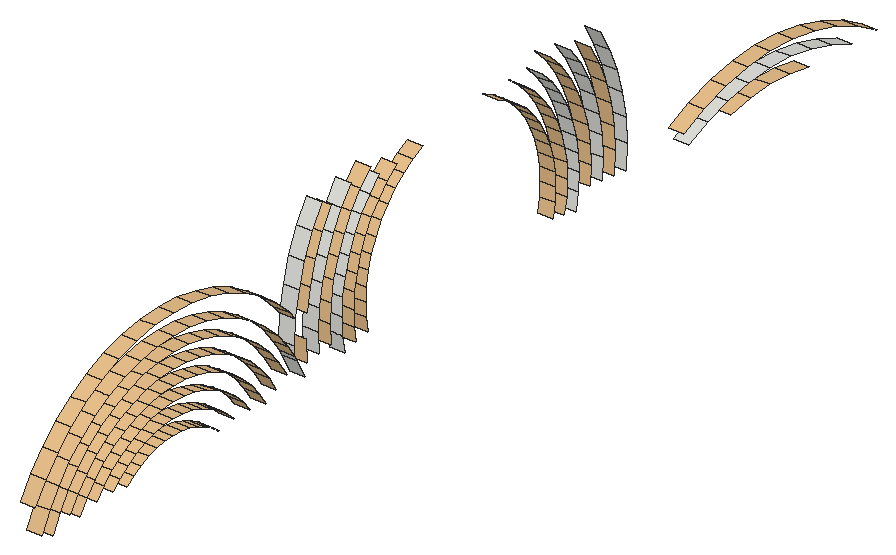
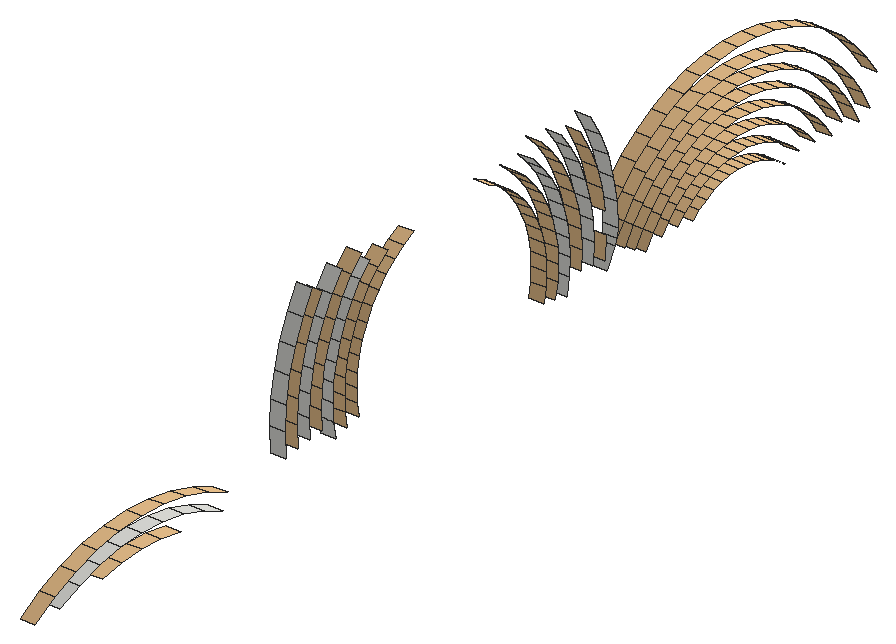
# SketchUp Ruby script. Lengths in inches.
U = 1.inch
M = Sketchup.active_model
def pt(a) = Geom::Point3d.new(a.map { |v| v * U })
def face(e, loops, mat)
  f = e.add_face(loops[0].map { |a| pt(a) })
  loops[1..].each { |l| e.add_face(l.map { |a| pt(a) }).erase! }
  f.material = f.back_material = mat if mat
  f
end
# faces: each face lists its corners as indices into pts; further lists are holes
def faces(e, pts, list, mat = nil) = list.each { |f| face(e, (f[0].is_a?(Array) ? f : [f]).map { |l| l.map { |i| pts[i] } }, mat) }
# xy, xz, yz: faces in a plane at the given z, y or x. An outline is a flat list of corners, or four numbers for a rectangle; further outlines are holes
def ring(l) = l.size == 4 ? [[l[0], l[1]], [l[2], l[1]], [l[2], l[3]], [l[0], l[3]]] : l.each_slice(2).to_a
def flat(e, list, mat, &to3) = list.each { |f| face(e, (f[0].is_a?(Array) ? f : [f]).map { |l| ring(l).map { |u, v| to3.(u, v) } }, mat) }
def xy(e, z, list, mat = nil) = flat(e, list, mat) { |x, y| [x, y, z] }
def xz(e, y, list, mat = nil) = flat(e, list, mat) { |x, z| [x, y, z] }
def yz(e, x, list, mat = nil) = flat(e, list, mat) { |y, z| [x, y, z] }
def lines(e, pts, list) = list.each { |a, b| e.add_line(pt(pts[a]), pt(pts[b])) }
# prism: a flat outline (further loops are holes) pulled along v
def prism(e, loops, v, mat = nil)
  f = face(e, loops, mat); d = Geom::Vector3d.new(v.map { |x| x * U })
  f.pushpull(f.normal.samedirection?(d) ? d.length : -d.length)
end
def box(e, o, s, mat = nil) = prism(e, [[o, [o[0] + s[0], o[1], o[2]], [o[0] + s[0], o[1] + s[1], o[2]], [o[0], o[1] + s[1], o[2]]]], [0, 0, s[2]], mat)
def at(x, y, z, deg = 0) = Geom::Transformation.translation(pt([x, y, z])) * Geom::Transformation.rotation(ORIGIN, Z_AXIS, deg.degrees)
def axes(o, x, y, z) = Geom::Transformation.new([*x, 0, *y, 0, *z, 0, *pt(o).to_a, 1])
def part(name) = M.definitions.add(name)
# library, detail: a bought-in or finely detailed component or shape, given as its bounding box
def library(name, o, s) = part(name).tap { |d| box(d.entities, o, s) }
def detail(e, o, s) = box(e.add_group.entities, o, s)
def put(e, d, t, mat = nil) = e.add_instance(d, t).tap { |i| i.material = mat if mat }
def group(e, t, mat = nil) = e.add_group.tap { |g| g.transformation = t; g.material = mat if mat }.entities
root = M.entities
M.materials.add("images").color = [235, 194, 141]
xz(root,90.53,[[183.82,66.87,185.82,66.88]])
p = [[183.82,51.02,60.88],[183.82,49.86,58.6],[185.82,49.86,58.6],[185.82,51.02,60.88],[183.82,85.65,58.71],[183.82,84.51,60.46],
  [185.82,84.51,60.46],[185.82,85.65,58.71],[183.82,156.61,58.71],[183.82,159.86,60.13],[185.82,159.86,60.13],[185.82,156.61,58.71],
  [183.82,188.1,58.8],[183.82,184.82,60.66],[185.82,184.82,60.66],[185.82,188.1,58.8],[183.82,55.64,60.6],[183.82,54.48,58.86],
  [185.82,54.48,58.86],[185.82,55.64,60.6],[183.82,76.66,59.78],[183.82,77.78,58.9375],[185.82,77.78,58.9375],[185.82,76.66,59.78],
  [183.82,180.68,60.25],[183.82,183.93,58.87],[185.82,183.93,58.87],[185.82,180.68,60.25],[183.82,62.35,59.01],[183.82,63.48,59.84],
  [185.82,63.48,59.84],[185.82,62.35,59.01],[183.82,98.47,61.31],[183.82,98.87,59.03],[185.82,98.87,59.03],[185.82,98.47,61.31],
  [183.82,137.66,58.97],[183.82,138.07,61.25],[185.82,138.07,61.25],[185.82,137.66,58.97],[183.82,90.86,61.68],[183.82,92.1,59.18],
  [185.82,92.1,59.18],[185.82,90.86,61.68],[183.82,166.97,59.8125],[183.82,163.71,59.22],[185.82,163.71,59.22],[185.82,166.97,59.8125],
  [183.82,80.25,59.34],[183.82,79.07,60.46],[185.82,79.07,60.46],[185.82,80.25,59.34],[183.82,81.71,60.71],[183.82,82.9,59.27],
  [185.82,82.9,59.27],[185.82,81.71,60.71],[183.82,176.83,59.3],[183.82,173.57,59.85],[185.82,173.57,59.85],[185.82,176.83,59.3],
  [183.82,48.03,59.4],[183.82,49.3,61.89],[185.82,49.3,61.89],[185.82,48.03,59.4],[183.82,57.23,59.4],[183.82,58.4375,60.82],
  [185.82,58.4375,60.82],[185.82,57.23,59.4],[183.82,61.07,60.55],[183.82,59.88,59.44],[185.82,59.88,59.44],[185.82,61.07,60.55],
  [183.82,136.08,61.49],[183.82,135.72,59.43],[185.82,135.72,59.43],[185.82,136.08,61.49],[183.82,100.8125,59.48],[183.82,100.45,61.54],
  [185.82,100.45,61.54],[185.82,100.8125,59.48],[183.82,86.12,61.65],[183.82,87.39,59.7],[185.82,87.39,59.7],[185.82,86.12,61.65],
  [183.82,64.6875,60.53],[185.82,64.6875,60.53],[183.82,75.46,60.48],[185.82,75.46,60.48],[183.82,170.27,60.03],[185.82,170.27,60.03],
  [183.82,52.75,59.87],[183.82,54.04,61.81],[185.82,54.04,61.81],[185.82,52.75,59.87],[183.82,102.44,61.77],[183.82,102.76,59.94],
  [185.82,102.76,59.94],[185.82,102.44,61.77],[183.82,133.77,59.9],[183.82,134.09,61.72],[185.82,134.09,61.72],[185.82,133.77,59.9],
  [183.82,163.24,61.16],[185.82,163.24,61.16],[183.82,146.01,60.31],[183.82,146.2,63.55],[185.82,146.2,63.55],[185.82,146.01,60.31],
  [183.82,177.28,61.25],[185.82,177.28,61.25],[183.82,65.97,61.08],[185.82,65.97,61.08],[183.82,74.18,61.04],[185.82,74.18,61.04],
  [183.82,77.77,61.44],[185.82,77.77,61.44],[183.82,83.17,62.07],[185.82,83.17,62.07],[183.82,144.2,63.56],[183.82,144.02,60.55],
  [185.82,144.02,60.55],[185.82,144.2,63.56],[183.82,159.16,62],[183.82,155.71,60.49],[185.82,155.71,60.49],[185.82,159.16,62],
  [183.82,56.99,62.2],[185.82,56.99,62.2],[183.82,62.39,61.52],[185.82,62.39,61.52],[183.82,92.51,60.62],[183.82,92.34,63.63],
  [185.82,92.34,63.63],[185.82,92.51,60.62],[183.82,80.37,61.99],[185.82,80.37,61.99],[183.82,89.13,60.6875],[183.82,87.73,62.83],
  [185.82,87.73,62.83],[185.82,89.13,60.6875],[183.82,181.35,62.14],[185.82,181.35,62.14],[183.82,59.8,62.09],[185.82,59.8,62.09],
  [183.82,142.04,60.78],[183.82,142.2,63.56],[185.82,142.2,63.56],[185.82,142.04,60.78],[183.82,52.4375,63.01],[185.82,52.4375,63.01],
  [183.82,94.34,63.63],[183.82,94.49,60.85],[185.82,94.49,60.85],[185.82,94.34,63.63],[183.82,72.85,61.45],[185.82,72.85,61.45],
  [183.82,140.2,63.5625],[183.82,140.05,61.02],[185.82,140.05,61.02],[185.82,140.2,63.5625],[183.82,67.3125,61.47],[185.82,67.3125,61.47],
  [183.82,96.48,61.08],[183.82,96.34,63.63],[185.82,96.34,63.63],[185.82,96.48,61.08],[183.82,166.72,61.8],[185.82,166.72,61.8],
  [183.82,173.79,61.84],[185.82,173.79,61.84],[183.82,98.34,63.625],[185.82,98.34,63.625],[183.82,138.2,63.56],[185.82,138.2,63.56],
  [183.82,71.47,61.69],[185.82,71.47,61.69],[183.82,76.37,62.26],[185.82,76.37,62.26],[183.82,63.8,62.32],[185.82,63.8,62.32],
  [183.82,68.6875,61.71],[185.82,68.6875,61.71],[183.82,100.34,63.62],[185.82,100.34,63.62],[183.82,136.2,63.57],[185.82,136.2,63.57],
  [183.82,84.64,63.4375],[185.82,84.64,63.4375],[183.82,70.08,61.78],[185.82,70.08,61.78],[183.82,90.41,62.38],[185.82,90.41,62.38],
  [183.82,134.2,63.57],[185.82,134.2,63.57],[183.82,55.54,63.58],[185.82,55.54,63.58],[183.82,102.34,63.62],[185.82,102.34,63.62],
  [183.82,170.25,62.03],[185.82,170.25,62.03],[183.82,50.84,64.21],[185.82,50.84,64.21],[183.82,78.88,63.11],[185.82,78.88,63.11],
  [183.82,162.77,63.11],[185.82,162.77,63.11],[183.82,61.29,63.19],[185.82,61.29,63.19],[183.82,81.66,63.51],[185.82,81.66,63.51],
  [183.82,177.73,63.2],[185.82,177.73,63.2],[183.82,58.52,63.63],[185.82,58.52,63.63],[183.82,65.3,62.96],[185.82,65.3,62.96],
  [183.82,74.875,62.91],[185.82,74.875,62.91],[183.82,89.34,64.02],[185.82,89.34,64.02],[183.82,90.34,63.64],[185.82,90.34,63.64],
  [183.82,86.1,64.8],[185.82,86.1,64.8],[183.82,73.32,63.39],[185.82,73.32,63.39],[183.82,54.09,64.96],[185.82,54.09,64.96],
  [183.82,66.86,63.42],[185.82,66.86,63.42],[183.82,77.27,64.05],[185.82,77.27,64.05],[183.82,166.48,63.78],[185.82,166.48,63.78],
  [183.82,62.91,64.12],[185.82,62.91,64.12],[183.82,174.01,63.83],[185.82,174.01,63.83],[183.82,48.65,65.86],[183.82,46.93,63.27],
  [185.82,46.93,63.27],[185.82,48.65,65.86],[183.82,68.46,63.7],[185.82,68.46,63.7],[183.82,71.71,63.68],[185.82,71.71,63.68],
  [183.82,82.95,65.04],[185.82,82.95,65.04],[183.82,79.99,64.77],[185.82,79.99,64.77],[183.82,57.24,65.17],[185.82,57.24,65.17],
  [183.82,60.2,64.87],[185.82,60.2,64.87],[183.82,90.53,66.87],[185.82,90.53,66.87],[183.82,94.5,66.41],[185.82,94.5,66.41],
  [183.82,96.49,66.17],[185.82,96.49,66.17],[183.82,98.47,65.9375],[185.82,98.47,65.9375],[183.82,100.46,65.7],[185.82,100.46,65.7],
  [183.82,102.45,65.47],[185.82,102.45,65.47],[183.82,134.1,65.42],[185.82,134.1,65.42],[183.82,136.09,65.65],[185.82,136.09,65.65],
  [183.82,138.07,65.88],[185.82,138.07,65.88],[183.82,140.06,66.11],[185.82,140.06,66.11],[183.82,142.05,66.34],[185.82,142.05,66.34],
  [183.82,144.03,66.57],[185.82,144.03,66.57],[183.82,146.02,66.8],[185.82,146.02,66.8],[183.82,70.09,63.78],[185.82,70.09,63.78],
  [183.82,170.24,64.03],[185.82,170.24,64.03],[183.82,75.57,64.79],[185.82,75.57,64.79],[183.82,87.56,66.17],[185.82,87.56,66.17],
  [183.82,64.62,64.84],[185.82,64.62,64.84],[183.82,52.65,66.34],[185.82,52.65,66.34],[183.82,66.41,65.37],[185.82,66.41,65.37],
  [183.82,73.79,65.33],[185.82,73.79,65.33],[183.82,78.18,65.83],[185.82,78.18,65.83],[183.82,84.25,66.57],[185.82,84.25,66.57],
  [183.82,62.02,65.91],[185.82,62.02,65.91],[183.82,55.96,66.71],[185.82,55.96,66.71],[183.82,81.09,66.4375],[185.82,81.09,66.4375],
  [183.82,59.11,66.55],[185.82,59.11,66.55],[183.82,71.96,65.67],[185.82,71.96,65.67],[183.82,68.24,65.68],[185.82,68.24,65.68],
  [183.82,133.78,67.25],[185.82,133.78,67.25],[183.82,102.77,67.29],[185.82,102.77,67.29],[183.82,135.73,67.7],[185.82,135.73,67.7],
  [183.82,70.1,65.78],[185.82,70.1,65.78],[183.82,100.83,67.76],[185.82,100.83,67.76],[183.82,76.26,66.67],[185.82,76.26,66.67],
  [183.82,50.66,68.23],[185.82,50.66,68.23],[183.82,63.95,66.73],[185.82,63.95,66.73],[183.82,98.88,68.22],[185.82,98.88,68.22],
  [183.82,137.67,68.16],[185.82,137.67,68.16],[183.82,139.62,68.62],[185.82,139.62,68.62],[183.82,85.54,68.09],[185.82,85.54,68.09],
  [183.82,96.94,68.68],[185.82,96.94,68.68],[183.82,54.68,68.24],[185.82,54.68,68.24],[183.82,141.57,69.08],[185.82,141.57,69.08],
  [183.82,79.08,67.61],[185.82,79.08,67.61],[183.82,94.99,69.15],[185.82,94.99,69.15],[183.82,61.13,67.7],[185.82,61.13,67.7],
  [183.82,82.2,68.1],[185.82,82.2,68.1],[183.82,92.52,66.64],[183.82,93.04,69.61],[185.82,93.04,69.61],[185.82,92.52,66.64],
  [183.82,143.51,69.54],[185.82,143.51,69.54],[183.82,58.02,68.22],[185.82,58.02,68.22],[183.82,65.96,67.32],[185.82,65.96,67.32],
  [183.82,74.26,67.28],[185.82,74.26,67.28],[183.82,145.46,70],[185.82,145.46,70],[183.82,89.56,68.04],[185.82,89.56,68.04],
  [183.82,91.1,70.08],[183.82,90.53,66.88],[185.82,90.53,66.88],[185.82,91.1,70.08],[183.82,133.25,69.02],[185.82,133.25,69.02],
  [183.82,68.02,67.67],[185.82,68.02,67.67],[183.82,72.2,67.65],[185.82,72.2,67.65],[183.82,103.31,69.07],[185.82,103.31,69.07],
  [183.82,76.95,68.54],[185.82,76.95,68.54],[183.82,63.27,68.61],[185.82,63.27,68.61],[183.82,70.11,67.78],[185.82,70.11,67.78],
  [183.82,135.13,69.7],[185.82,135.13,69.7],[183.82,101.43,69.75],[185.82,101.43,69.75],[183.82,87.31,70.18],[185.82,87.31,70.18],
  [183.82,79.99,69.39],[185.82,79.99,69.39],[183.82,83.31,69.77],[185.82,83.31,69.77],[183.82,52.94,70.35],[185.82,52.94,70.35],
  [183.82,56.93,69.9],[185.82,56.93,69.9],[183.82,60.24,69.49],[185.82,60.24,69.49],[183.82,99.55,70.44],[185.82,99.55,70.44],
  [183.82,137.01,70.38],[185.82,137.01,70.38],[183.82,74.73,69.22],[185.82,74.73,69.22],[183.82,65.5,69.27],[185.82,65.5,69.27],
  [183.82,138.89,71.07],[185.82,138.89,71.07],[183.82,97.67,71.13],[185.82,97.67,71.13],[183.82,132.52,70.72],[185.82,132.52,70.72],
  [183.82,95.79,71.8125],[185.82,95.79,71.8125],[183.82,104.04,70.77],[185.82,104.04,70.77],[183.82,140.77,71.75],[185.82,140.77,71.75],
  [183.82,72.44,69.64],[185.82,72.44,69.64],[183.82,67.8,69.66],[185.82,67.8,69.66],[183.82,77.65,70.42],[185.82,77.65,70.42],
  [183.82,62.6,70.49],[185.82,62.6,70.49],[183.82,142.65,72.43],[185.82,142.65,72.43],[183.82,70.12,69.78],[185.82,70.12,69.78],
  [183.82,93.91,72.5],[185.82,93.91,72.5],[183.82,134.31,71.62],[185.82,134.31,71.62],[183.82,80.9,71.18],[185.82,80.9,71.18],
  [183.82,102.26,71.67],[185.82,102.26,71.67],[183.82,59.36,71.28],[185.82,59.36,71.28],[183.82,144.53,73.11],[185.82,144.53,73.11],
  [183.82,92.04,73.1875],[185.82,92.04,73.1875],[183.82,84.82,72.05],[185.82,84.82,72.05],[183.82,55.4375,72.19],[185.82,55.4375,72.19],
  [183.82,75.2,71.16],[185.82,75.2,71.16],[183.82,100.47,72.57],[185.82,100.47,72.57],[183.82,136.1,72.51],[185.82,136.1,72.51],
  [183.82,65.05,71.21],[185.82,65.05,71.21],[183.82,131.6,72.33],[185.82,131.6,72.33],[183.82,104.97,72.37],[185.82,104.97,72.37],
  [183.82,98.68,73.47],[185.82,98.68,73.47],[183.82,137.89,73.41],[185.82,137.89,73.41],[183.82,67.57,71.65],[185.82,67.57,71.65],
  [183.82,72.68,71.62],[185.82,72.68,71.62],[183.82,78.34,72.29],[185.82,78.34,72.29],[183.82,61.92,72.375],[185.82,61.92,72.375],
  [183.82,70.13,71.78],[185.82,70.13,71.78],[183.82,133.27,73.43],[185.82,133.27,73.43],[183.82,103.3,73.47],[185.82,103.3,73.47],
  [183.82,139.68,74.3],[185.82,139.68,74.3],[183.82,96.9,74.37],[185.82,96.9,74.37],[183.82,82.14,73.62],[185.82,82.14,73.62],
  [183.82,58.14,73.74],[185.82,58.14,73.74],[183.82,75.67,73.11],[185.82,75.67,73.11],[183.82,130.49,73.82],[185.82,130.49,73.82],
  [183.82,64.6,73.16],[185.82,64.6,73.16],[183.82,106.08,73.86],[185.82,106.08,73.86],[183.82,141.46,75.2],[185.82,141.46,75.2],
  [183.82,95.11,75.27],[185.82,95.11,75.27],[183.82,134.94,74.52],[185.82,134.94,74.52],[183.82,101.63,74.57],[185.82,101.63,74.57],
  [183.82,72.92,73.61],[185.82,72.92,73.61],[183.82,143.25,76.09],[185.82,143.25,76.09],[183.82,67.35,73.63],[185.82,67.35,73.63],
  [183.82,93.33,76.17],[185.82,93.33,76.17],[183.82,132.03,75.1],[185.82,132.03,75.1],[183.82,136.61,75.62],[185.82,136.61,75.62],
  [183.82,99.96,75.67],[185.82,99.96,75.67],[183.82,104.55,75.14],[185.82,104.55,75.14],[183.82,70.14,73.78],[185.82,70.14,73.78],
  [183.82,79.29,74.86],[185.82,79.29,74.86],[183.82,61,74.95],[185.82,61,74.95],[183.82,129.22,75.17],[185.82,129.22,75.17],
  [183.82,107.35,75.2],[185.82,107.35,75.2],[183.82,138.29,76.72],[185.82,138.29,76.72],[183.82,98.29,76.78],[185.82,98.29,76.78],
  [183.82,133.56,76.39],[185.82,133.56,76.39],[183.82,103.02,76.43],[185.82,103.02,76.43],[183.82,76.32,75.77],[185.82,76.32,75.77],
  [183.82,63.98,75.83],[185.82,63.98,75.83],[183.82,105.98,76.66],[185.82,105.98,76.66],[183.82,130.6,76.62],[185.82,130.6,76.62],
  [183.82,108.77,76.39],[185.82,108.77,76.39],[183.82,127.81,76.36],[185.82,127.81,76.36],[183.82,139.96,77.8125],[185.82,139.96,77.8125],
  [183.82,96.625,77.88],[185.82,96.625,77.88],[183.82,135.09,77.67],[185.82,135.09,77.67],[183.82,101.49,77.72],[185.82,101.49,77.72],
  [183.82,67.05,76.36],[185.82,67.05,76.36],[183.82,73.26,76.32],[185.82,73.26,76.32],[183.82,141.63,78.91],[185.82,141.63,78.91],
  [183.82,94.95,78.98],[185.82,94.95,78.98],[183.82,70.15,76.52],[185.82,70.15,76.52],[183.82,104.61,78.11],[185.82,104.61,78.11],
  [183.82,110.32,77.41],[185.82,110.32,77.41],[183.82,126.26,77.38],[185.82,126.26,77.38],[183.82,131.97,78.07],[185.82,131.97,78.07],
  [183.82,129,77.96],[185.82,129,77.96],[183.82,107.58,78],[185.82,107.58,78],[183.82,136.63,78.95],[185.82,136.63,78.95],
  [183.82,99.96,79.01],[185.82,99.96,79.01],[183.82,111.98,78.24],[185.82,111.98,78.24],[183.82,124.6,78.22],[185.82,124.6,78.22],
  [183.82,103.24,79.57],[185.82,103.24,79.57],[183.82,133.35,79.53],[185.82,133.35,79.53]]
faces(root,p,[[0,1,2,3],[4,5,6,7],[12,13,14,15],[16,17,18,19],[20,21,22,23],[28,29,30,31],[44,45,46,47],[48,49,50,51],
  [52,53,54,55],[56,57,58,59],[60,61,62,63],[64,65,66,67],[68,69,70,71],[72,73,74,75],[76,77,78,79],[80,81,82,83],
  [29,84,85,30],[86,20,23,87],[88,44,47,89],[90,91,92,93],[94,95,96,97],[98,99,100,101],[57,88,89,58],[84,110,111,85],
  [112,86,87,113],[49,114,115,50],[5,116,117,6],[118,119,120,121],[122,123,124,125],[126,16,19,127],[128,68,71,129],[130,131,132,133],
  [134,52,55,135],[136,137,138,139],[13,140,141,14],[65,142,143,66],[148,0,3,149],[154,112,113,155],[156,157,158,159],[110,160,161,111],
  [162,163,164,165],[174,154,155,175],[114,176,177,115],[178,128,129,179],[160,180,181,161],[77,182,183,78],[184,72,75,185],[186,80,83,187],
  [180,188,189,181],[188,174,175,189],[99,192,193,100],[91,194,195,92],[196,94,97,197],[61,200,201,62],[202,134,135,203],[204,122,125,205],
  [142,206,207,143],[116,208,209,117],[140,210,211,141],[212,126,127,213],[214,178,179,215],[176,216,217,177],[218,190,191,219],[137,222,223,138],
  [216,224,225,217],[226,148,149,227],[228,214,215,229],[230,202,203,231],[232,204,205,233],[206,234,235,207],[210,236,237,211],[238,239,240,241],
  [242,228,229,243],[224,244,245,225],[246,186,187,247],[208,248,249,209],[194,250,251,195],[252,212,213,253],[163,258,259,164],[182,262,263,183],
  [264,196,197,265],[192,266,267,193],[268,184,185,269],[272,156,159,273],[276,118,121,277],[280,242,243,281],[244,280,281,245],[282,232,233,283],
  [236,282,283,237],[284,230,231,285],[286,218,219,287],[234,288,289,235],[200,290,291,201],[288,292,293,289],[294,284,285,295],[248,296,297,249],
  [222,298,299,223],[300,252,253,301],[302,226,227,303],[304,246,247,305],[250,306,307,251],[308,294,295,309],[292,310,311,293],[266,312,313,267],
  [314,264,265,315],[316,268,269,317],[310,318,319,311],[318,308,309,319],[262,320,321,263],[296,322,323,297],[324,238,241,325],[326,300,301,327],
  [332,272,273,333],[334,286,287,335],[258,336,337,259],[290,338,339,291],[342,304,305,343],[306,346,347,307],[298,348,349,299],[350,351,352,353],
  [354,276,277,355],[356,302,303,357],[358,326,327,359],[322,360,361,323],[254,364,365,255],[312,370,371,313],[372,358,359,373],[360,374,375,361],
  [376,314,315,377],[378,342,343,379],[346,380,381,347],[382,372,373,383],[374,382,383,375],[384,316,317,385],[320,386,387,321],[364,388,389,365],
  [348,390,391,349],[392,334,335,393],[394,324,325,395],[338,396,397,339],[398,356,357,399],[404,378,379,405],[380,406,407,381],[408,332,333,409],
  [336,410,411,337],[370,412,413,371],[416,376,377,417],[420,404,405,421],[406,422,423,407],[390,424,425,391],[426,398,399,427],[428,354,355,429],
  [430,420,421,431],[351,432,433,352],[422,430,431,423],[434,384,385,435],[436,392,393,437],[386,438,439,387],[396,440,441,397],[388,446,447,389],
  [448,394,395,449],[424,450,451,425],[456,426,427,457],[412,458,459,413],[460,416,417,461],[410,462,463,411],[464,408,409,465],[466,456,457,467],
  [450,468,469,451],[470,436,437,471],[440,472,473,441],[474,466,467,475],[468,474,475,469],[476,434,435,477],[438,478,479,439],[446,484,485,447],
  [486,448,449,487],[488,470,471,489],[458,490,491,459],[472,492,493,473],[494,460,461,495],[496,428,429,497],[432,498,499,433],[504,488,489,505],
  [492,508,509,493],[512,476,477,513],[514,464,465,515],[462,516,517,463],[478,518,519,479],[508,520,521,509],[520,504,505,521],[484,522,523,485],
  [524,486,487,525],[490,526,527,491],[528,494,495,529],[522,538,539,523],[540,524,525,541],[518,542,543,519],[544,512,513,545],[546,528,529,547],
  [526,548,549,527],[550,496,497,551],[498,552,553,499],[554,514,515,555],[516,556,557,517],[558,540,541,559],[538,560,561,539],[560,566,567,561],
  [566,558,559,567],[570,546,547,571],[548,572,573,549],[576,544,545,577],[542,578,579,543],[584,570,571,585],[572,586,587,573],[556,588,589,557],
  [590,554,555,591]],"images")
faces(root,p,[[8,9,10,11],[24,25,26,27],[32,33,34,35],[36,37,38,39],[40,41,42,43],[9,102,103,10],[104,105,106,107],[108,24,27,109],
  [144,145,146,147],[150,151,152,153],[102,166,167,103],[168,108,109,169],[170,32,35,171],[37,172,173,38],[190,40,43,191],[166,198,199,167],
  [198,168,169,199],[220,190,191,221],[254,220,221,255],[256,150,153,257],[260,170,171,261],[172,270,271,173],[145,274,275,146],[105,278,279,106],
  [328,260,261,329],[270,330,331,271],[274,340,341,275],[344,256,257,345],[278,362,363,279],[366,367,368,369],[400,328,329,401],[330,402,403,331],
  [414,344,345,415],[340,418,419,341],[362,442,443,363],[444,366,369,445],[452,400,401,453],[402,454,455,403],[418,480,481,419],[482,414,415,483],
  [454,500,501,455],[502,452,453,503],[442,506,507,443],[510,444,445,511],[480,530,531,481],[532,482,483,533],[500,534,535,501],[536,502,503,537],
  [506,562,563,507],[564,510,511,565],[568,536,537,569],[534,574,575,535],[530,580,581,531],[582,532,533,583]])
